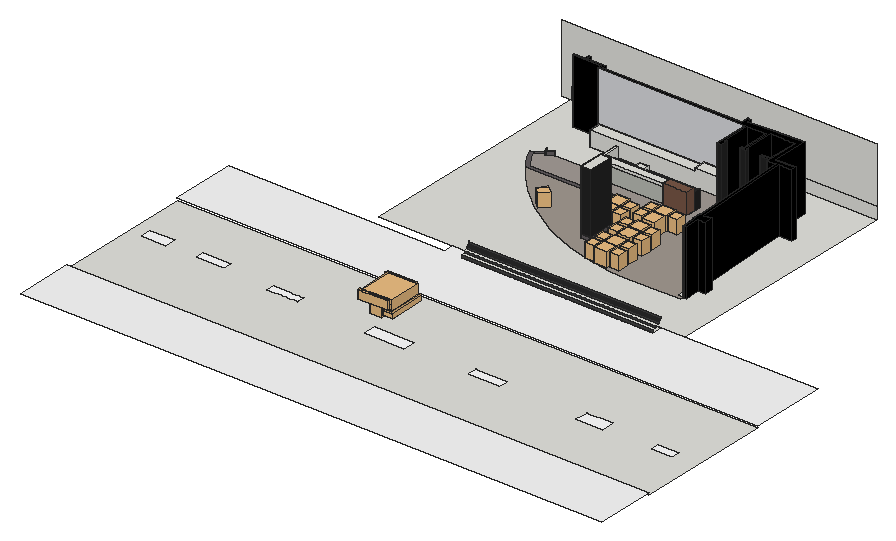
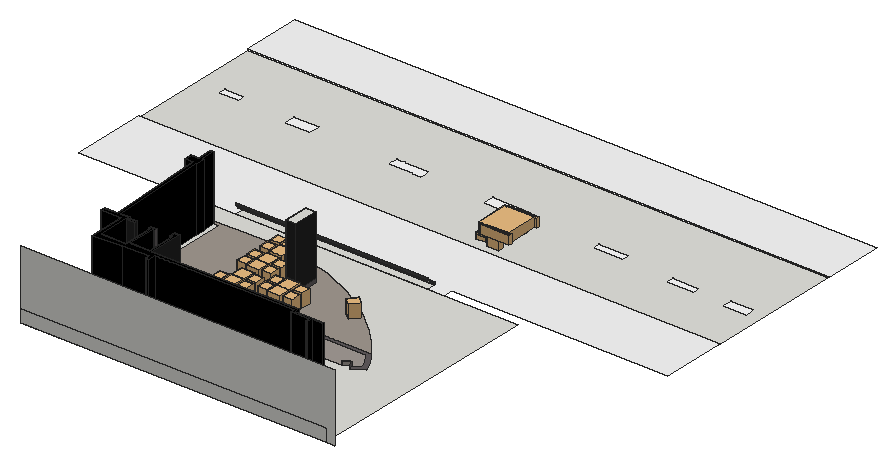
# SketchUp Ruby script. Lengths in inches.
U = 1.inch
M = Sketchup.active_model
def pt(a) = Geom::Point3d.new(a.map { |v| v * U })
def face(e, loops, mat)
  f = e.add_face(loops[0].map { |a| pt(a) })
  loops[1..].each { |l| e.add_face(l.map { |a| pt(a) }).erase! }
  f.material = f.back_material = mat if mat
  f
end
# faces: each face lists its corners as indices into pts; further lists are holes
def faces(e, pts, list, mat = nil) = list.each { |f| face(e, (f[0].is_a?(Array) ? f : [f]).map { |l| l.map { |i| pts[i] } }, mat) }
# xy, xz, yz: faces in a plane at the given z, y or x. An outline is a flat list of corners, or four numbers for a rectangle; further outlines are holes
def ring(l) = l.size == 4 ? [[l[0], l[1]], [l[2], l[1]], [l[2], l[3]], [l[0], l[3]]] : l.each_slice(2).to_a
def flat(e, list, mat, &to3) = list.each { |f| face(e, (f[0].is_a?(Array) ? f : [f]).map { |l| ring(l).map { |u, v| to3.(u, v) } }, mat) }
def xy(e, z, list, mat = nil) = flat(e, list, mat) { |x, y| [x, y, z] }
def xz(e, y, list, mat = nil) = flat(e, list, mat) { |x, z| [x, y, z] }
def yz(e, x, list, mat = nil) = flat(e, list, mat) { |y, z| [x, y, z] }
def lines(e, pts, list) = list.each { |a, b| e.add_line(pt(pts[a]), pt(pts[b])) }
# prism: a flat outline (further loops are holes) pulled along v
def prism(e, loops, v, mat = nil)
  f = face(e, loops, mat); d = Geom::Vector3d.new(v.map { |x| x * U })
  f.pushpull(f.normal.samedirection?(d) ? d.length : -d.length)
end
def box(e, o, s, mat = nil) = prism(e, [[o, [o[0] + s[0], o[1], o[2]], [o[0] + s[0], o[1] + s[1], o[2]], [o[0], o[1] + s[1], o[2]]]], [0, 0, s[2]], mat)
def at(x, y, z, deg = 0) = Geom::Transformation.translation(pt([x, y, z])) * Geom::Transformation.rotation(ORIGIN, Z_AXIS, deg.degrees)
def axes(o, x, y, z) = Geom::Transformation.new([*x, 0, *y, 0, *z, 0, *pt(o).to_a, 1])
def part(name) = M.definitions.add(name)
# library, detail: a bought-in or finely detailed component or shape, given as its bounding box
def library(name, o, s) = part(name).tap { |d| box(d.entities, o, s) }
def detail(e, o, s) = box(e.add_group.entities, o, s)
def put(e, d, t, mat = nil) = e.add_instance(d, t).tap { |i| i.material = mat if mat }
def group(e, t, mat = nil) = e.add_group.tap { |g| g.transformation = t; g.material = mat if mat }.entities
root = M.entities
M.materials.add("Biselado").color = [218, 219, 223]
M.materials.add("Color_").color = [255, 255, 255]
M.materials.add("Concrete").color = [186, 188, 181]
M.materials.add("Floor board2").color = [119, 86, 70]
M.materials.add("Plastic Black ").color = [43, 43, 43]
M.materials.add("Screen Shot 2014-10-30 at 12.13.07").color = [162, 155, 149]
M.materials.add("Sophie_Shoes2").color = [35, 35, 35]
M.materials.add("Sophie_Skirt").color = [0, 0, 0]
M.materials.add("Stain").color = [141, 140, 139]
M.materials.add("Untitsled-1").color = [96, 91, 93]
M.materials.add("Wood_Grain_Dark").color = [51, 47, 43]
M.materials.add("[0132_LightGray]").color = [169, 169, 169]
M.materials.add("[Color_000]").color = [255, 255, 255]
M.materials.add("[Granite Dark Gray]").color = [69, 68, 68]
M.materials.add("[Tile Grey]").color = [249, 249, 249]
M.materials.add("s500 white").color = [237, 237, 230]
M.materials.add("s600").color = [22, 22, 22]
M.materials.add("t_planksnew0027_5_l_seamless_298 copy").color = [161, 153, 144]
c1 = library("Group\#661",[0,74.4,0],[63.33,6.34,17.85])
c2 = library("Car wheel",[-30.53,-13.73,-29.67],[182.47,72.82,182.83])
c3 = library("Group\#641",[0,0,0],[63.89,71.13,20.26])
c4 = library("ch24 wishbone chair by Carl Hansen & Son",[0,0,0],[21.1,19.68,29.02])
c5 = part("Group\#651")
p = [[17.05,0,0.12],[10.76,0.83,0.14],[10.77,0.78,0],[8.125,1.26,0.14],[7.82,1.25,0],[5.66,2.14,0],
  [5.93,2.16,0.13],[4.78,3.14,0.17],[4.32,3.23,0],[3.41,4.89,0],[3.73,4.98,0.17],[1.67,12.39,0],
  [2,12.39,0.17],[0,22.05,0],[0.34,21.8125,0.17],[1.49,22.05,0.22],[16.1,0.375,0.31],[17.15,0.01,0.31],
  [14.125,0.92,0.31],[11.23,1.28,0.31],[8.51,1.62,0.31],[5.54,2.89,0.31],[5.22,3.53,0.31],[4.82,5.07,0.31],
  [3.125,12.39,0.31],[1.65,21.85,0.31]]
faces(c5.entities,p,[[0,1,2],[2,3,4],[3,2,1],[5,4,6],[6,4,3],[7,8,5],[7,5,6],[9,7,10],
  [7,9,8],[11,9,12],[12,9,10],[13,11,14],[14,11,12],[14,15,13],[16,1,17],[1,0,17],
  [1,16,18],[19,3,1],[19,1,18],[3,20,6],[3,19,20],[6,20,21],[21,7,6],[22,7,21],
  [10,7,23],[22,23,7],[24,12,10],[23,24,10],[14,12,25],[24,25,12],[14,25,15]],"[0132_LightGray]")
c6 = library("Component\#54",[-0.14,0,-0.04],[12.61,20.03,8.76])
c7 = library("Group\#643",[0,0,0],[21.93,78.33,4.58])
c8 = library("Group\#650",[0,0,0],[20.12,77.4,9.12])
c9 = library("Group\#658",[0,0,0],[7.9,66.99,3.86])
c10 = part("Untitled (5)")
xy(c10.entities,0,[[[158.81,26.5625,306.06,993.3125],[226.57,518.17,239.57,583.92],[225.28,357.51,237.28,411.51],[222.61,182.28,236.36,226.53],[239.71,931.55,251.46,972.3],[233.64,703.93,242.14,755.18],[240.05,835.03,248.8,880.53],[222.04,66.5,231.29,100.5]]])
xy(c10.entities,0,[[222.04,66.5,231.29,100.5],[222.61,182.28,236.36,226.53],[225.28,357.51,237.28,411.51],[226.57,518.17,239.57,583.92],[233.64,703.93,242.14,755.18],
  [240.05,835.03,248.8,880.53],[239.71,931.55,251.46,972.3]],"Color_")
c11 = library("Square table",[5.01,5.91,-0.2],[27.56,27.56,29.53])
xy(root,-20.5,[[3028.45,559.875,3440.34,581.125],[2834.69,581.125,3491.44,1096.5]])
xy(root,-20.5,[[2527.87,419.4375,3778.5,419.4375,3778.5,581.125,3440.34,581.125,3440.34,559.875,3028.45,559.875,3028.45,581.125,2993.46,581.125,2993.46,559.875,2527.87,559.875]],"[Tile Grey]")
xy(root,-20.25,[[2527.87,0,3778.5,126.25]],"[Tile Grey]")
xy(root,-15.38,[[3028.45,559.875,3440.34,568.25]])
xy(root,-10.73,[[3028.45,568.25,3440.34,575.4375]])
xy(root,-6.62,[[3028.45,575.4375,3440.34,578]])
xy(root,-3.61,[[3028.45,578,3440.34,580.3125]])
xz(root,559.875,[[3028.45,-20.5,3440.34,-15.38]],"[Granite Dark Gray]")
xz(root,568.25,[[3028.45,-15.38,3440.34,-10.73]],"[Granite Dark Gray]")
xz(root,575.4375,[[3028.45,-10.73,3440.34,-6.62]],"[Granite Dark Gray]")
xz(root,578,[[3028.45,-6.62,3440.34,-3.61]],"[Granite Dark Gray]")
xz(root,580.3125,[[3028.45,-3.61,3440.34,1.19]],"[Granite Dark Gray]")
xz(root,1096.5,[[2814.94,-20.5,2814.94,126,3491.44,126,3491.44,6,2834.69,6,2834.69,-20.5],[2834.69,-20.5,3491.44,6]])
yz(root,3028.45,[[578,-6.62,581.125,-3.61],[580.3125,-3.61,581.125,1.19]])
p = [[3061.4375,322.92,0.24],[3061.4375,322.92,0.29],[3037.61,365.74,-9.8],[3037.48,365.73,-9.67],[3037.1875,403.93,-9.8],[3037.05,403.92,-9.67]]
lines(root,p,[[0,1],[2,3],[4,5]])
put(root,c1,axes([3062.39,318.93,-4.37],[-0.99994,-0.01119,0],[-0.01119,0.99994,0],[0,0,1]))
put(root,c1,at(3061.49,399.66,-4.37,-179.359))
put(root,c2,axes([3043.5,395.9,-19.76],[-0.14272,-0.0016,0],[0.0018,-0.16111,0],[0,0,0.14273]))
put(root,c2,axes([3044.33,322.28,-19.76],[-0.14272,-0.0016,0],[-0.0018,0.16111,0],[0,0,0.14273]))
put(root,c3,at(3067.45,394.92,-5.53,-179.359))
put(root,c4,axes([3031.75,755.79,0],[0.63382,0.77348,0],[0.77348,-0.63382,0],[0,0,1]))
put(root,c5,at(3066.33,398.45,-4.68,-179.359),"s600")
put(root,c6,at(3064.43,397.01,-3.93,-179.359))
put(root,c5,axes([3067.2,320.25,-4.68],[-0.99994,-0.01119,0],[-0.01119,0.99994,0],[0,0,1]),"s600")
put(root,c6,axes([3065.27,321.65,-3.93],[-0.99994,-0.01119,0],[-0.01119,0.99994,0],[0,0,1]))
put(root,c7,at(3070.37,398.56,-8.95,-179.359))
put(root,c8,at(3070.4375,398.09,-18.05,-179.359),"s600")
g1 = group(root,at(3064.73,393.36,-4.37,-179.359))
p = [[1.7,7.17,1.16],[1.47,7.32,0],[3.4,0,1.16],[3.17,0,0],[0.28,16.38,1.16],[0,16.77,0],
  [0.28,51.68,1.16],[1.47,60.75,0],[0,51.29,0],[1.7,60.89,1.16],[3.4,68.07,1.16],[3.17,68.06,0]]
faces(g1,p,[[0,1,2],[3,2,1],[4,1,0],[1,4,5],[6,7,8],[7,6,9],[7,9,10],[10,11,7]],"s500 white")
put(root,c9,at(3069.3125,392.875,-15.46,-179.359),"s600")
g2 = group(root,at(3122.24,896.18,31.5))
xy(g2,-31.5,[[0,19.69,18.11,26.38]])
xy(g2,0,[[[0,0,18.11,19.69],[1.09,8.35,17.09,13.35]]])
xy(g2,3.9375,[[[0,0,18.11,26.38],[1.09,8.35,17.09,13.35]]])
xz(g2,0,[[0,0,18.11,3.9375]])
xz(g2,8.35,[[1.09,0,17.09,3.9375]])
xz(g2,13.35,[[1.09,0,17.09,3.9375]])
xz(g2,19.69,[[0,-31.5,18.11,0]])
xz(g2,26.38,[[0,-31.5,18.11,3.9375]])
yz(g2,0,[[19.69,-31.5,19.69,0,0,0,0,3.9375,26.38,3.9375,26.38,-31.5]])
yz(g2,1.09,[[8.35,0,13.35,3.9375]])
yz(g2,17.09,[[8.35,0,13.35,3.9375]])
yz(g2,18.11,[[19.69,-31.5,26.38,-31.5,26.38,3.9375,0,3.9375,0,0,19.69,0]])
g3 = group(root,at(2791.37,624.35,0))
xy(g3,0,[[190.59,338.75,502.63,364.34]],"Stain")
xy(g3,31.5,[[190.59,338.75,416.02,364.34]])
xy(g3,37.4,[[416.02,338.75,502.63,364.34]])
xz(g3,338.75,[[190.59,0,502.63,0,502.63,37.4,416.02,37.4,416.02,31.5,190.59,31.5]])
xz(g3,364.34,[[190.59,0,190.59,31.5,416.02,31.5,416.02,37.4,502.63,37.4,502.63,0]],"Stain")
yz(g3,190.59,[[338.75,0,364.34,31.5]],"Stain")
yz(g3,416.02,[[338.75,31.5,364.34,37.4]])
yz(g3,502.63,[[338.75,0,364.34,37.4]],"Stain")
put(root,c4,axes([3149.53,792.13,0],[0.00287,-1,0],[-1,-0.00287,0],[0,0,1]))
put(root,c4,axes([3149.53,819.14,0],[0.00287,-1,0],[-1,-0.00287,0],[0,0,1]))
g4 = group(root,at(3074.02,896.18,0))
g5 = group(g4,at(0,0,0))
box(g5,[-5.91,0,0],[163.69,19.69,31.5])
put(root,c10,axes([3812.77,-189.95,-24.3125],[0,1.99109,0],[-1.29,0,0],[0,0,1.29]))
g6 = group(root,at(2911.82,841.06,0),"Untitsled-1")
xy(g6,0,[[30.66,0,22.97,10.41,13.17,25.17,0,47.23,25.07,61.99,28.66,54.97,10.82,44.46,19.84,29.37,29.42,14.93,34.63,7.875,502.55,7.875,502.55,0],[29.6875,52.96,28.66,54.97,25.07,61.99,25.45,62.21,29.03,55.19,29.87,53.55,30.06,53.17],[150.39,55.12,162.2,61.02]])
xy(g6,0,[[34.63,7.875,29.42,14.93,19.84,29.37,10.82,44.46,28.66,54.97,29.6875,52.96,30.06,53.17,43.36,60.59,43.25,60.59,43.25,61.02,150.39,61.02,150.39,55.12,295.57,55.12,295.57,74.8,303.44,74.8,303.44,147.64,382.18,147.64,382.18,74.8,392.39,74.8,392.39,88.58,388.09,88.58,388.09,147.64,428.18,147.64,428.18,88.58,423.88,88.58,423.88,82.68,436.24,82.68,436.24,88.58,434.09,88.58,434.09,153.54,485.64,153.54,485.64,88.58,467.74,88.58,467.74,82.68,480.91,82.68,480.91,79.03,503.34,79.03,503.34,31.5,502.55,31.5,502.55,7.875]],"Screen Shot 2014-10-30 at 12.13.07")
xy(g6,0,[[295.57,74.8,303.44,147.64]],"Untitsled-1")
xy(g6,7.875,[[29.6875,52.96,25.07,61.99,25.45,62.21,29.03,55.19,29.87,53.55,43.25,61.02,43.25,60.59,43.36,60.59]],"Untitsled-1")
xz(g6,60.59,[[43.25,0,43.36,7.875]],"Screen Shot 2014-10-30 at 12.13.07")
yz(g6,43.25,[[60.59,0,61.02,7.875]],"Screen Shot 2014-10-30 at 12.13.07")
p = [[29.6875,52.96,7.875],[25.07,61.99,7.875],[25.07,61.99,0],[28.66,54.97,0],[29.6875,52.96,0],[30.06,53.17,0],
  [43.36,60.59,0],[43.36,60.59,7.875],[29.87,53.55,0],[29.03,55.19,0],[29.03,55.19,7.875],[29.87,53.55,7.875],
  [43.25,61.02,0],[43.25,61.02,7.875],[25.45,62.21,0],[25.45,62.21,7.875],[150.39,55.12,0],[150.39,39.37,0],
  [502.55,0,0],[503.34,0,0],[29.44,55.42,0],[43.45,60.64,0],[25.07,62,0],[502.55,78.21,0],
  [480.91,78.21,0],[480.91,79.03,0],[303.44,147.64,0],[303.44,155.51,0]]
faces(g6,p,[[0,1,2,3,4],[4,5,6,7,0],[8,9,10,11],[9,14,15,10],[14,2,1,15]])
faces(g6,p,[[8,12,13,11]],"Screen Shot 2014-10-30 at 12.13.07")
lines(g6,p,[[16,17],[18,19],[20,9],[6,21],[22,2],[23,24],[24,25],[26,27]])
g7 = group(g6,at(388.09,147.64,0))
xy(g7,0,[[0,-59.06,4.3,-59.06,4.3,-58.62,0.43,-58.62,0.43,-0.43,39.67,-0.43,39.67,-58.62,35.8,-58.62,35.8,-59.06,40.1,-59.06,40.1,0,0,0]],"Screen Shot 2014-10-30 at 12.13.07")
xy(g7,7.875,[[0,-59.06,0,-0.43,0.43,-0.43,0.43,-58.62,4.3,-58.62,4.3,-59.06],[35.8,-59.06,35.8,-58.62,39.67,-58.62,39.67,-0.43,40.1,-0.43,40.1,-59.06]],"Untitsled-1")
xy(g7,47.24,[[0,-0.43,40.1,0]],"Untitsled-1")
xz(g7,-59.06,[[35.8,0,40.1,7.875]],"Screen Shot 2014-10-30 at 12.13.07")
xz(g7,-59.06,[[0,0,4.3,7.875]],"Untitsled-1")
xz(g7,-58.62,[[0.43,0,4.3,7.875],[35.8,0,39.67,7.875]],"Untitsled-1")
xz(g7,-0.43,[[0,7.875,40.1,39.37]],"Screen Shot 2014-10-30 at 12.13.07")
xz(g7,-0.43,[[0.43,0,39.67,7.875],[0,39.37,40.1,47.24]],"Untitsled-1")
yz(g7,0,[[-59.06,0,0,0,0,39.37,-0.43,39.37,-0.43,7.875,-59.06,7.875]],"Screen Shot 2014-10-30 at 12.13.07")
yz(g7,0,[[-0.43,39.37,0,47.24]],"Untitsled-1")
yz(g7,0.43,[[-58.62,0,-0.43,7.875]],"Untitsled-1")
yz(g7,4.3,[[-59.06,0,-58.62,7.875]],"Untitsled-1")
yz(g7,35.8,[[-59.06,0,-58.62,7.875]],"Untitsled-1")
yz(g7,39.67,[[-58.62,0,-0.43,7.875]],"Untitsled-1")
yz(g7,40.1,[[-59.06,0,-59.06,7.875,-0.43,7.875,-0.43,39.37,0,39.37,0,0]],"Screen Shot 2014-10-30 at 12.13.07")
yz(g7,40.1,[[-0.43,39.37,0,47.24]],"Untitsled-1")
g8 = group(g6,at(434.09,153.54,0))
xy(g8,0,[[0,-64.96,2.15,-64.96,2.15,-64.53,0.43,-64.53,0.43,-0.43,51.11,-0.43,51.11,-64.53,33.65,-64.53,33.65,-64.96,51.55,-64.96,51.55,0,0,0]],"Screen Shot 2014-10-30 at 12.13.07")
xy(g8,7.875,[[0,-64.96,0,-0.43,0.43,-0.43,0.43,-64.53,2.15,-64.53,2.15,-64.96],[33.65,-64.96,33.65,-64.53,51.11,-64.53,51.11,-0.43,51.55,-0.43,51.55,-64.96]],"Untitsled-1")
xy(g8,47.24,[[0,-0.43,51.55,0]],"Untitsled-1")
xz(g8,-64.96,[[0,0,2.15,7.875],[33.65,0,51.55,7.875]],"Untitsled-1")
xz(g8,-64.53,[[0.43,0,2.15,7.875],[33.65,0,51.11,7.875]],"Untitsled-1")
xz(g8,-0.43,[[0,7.875,51.55,39.37]],"Screen Shot 2014-10-30 at 12.13.07")
xz(g8,-0.43,[[0.43,0,51.11,7.875],[0,39.37,51.55,47.24]],"Untitsled-1")
xz(g8,0,[[40.1,0,51.55,39.37]],"Screen Shot 2014-10-30 at 12.13.07")
xz(g8,0,[[40.1,39.37,51.55,47.24]],"Untitsled-1")
yz(g8,0,[[-64.96,0,0,0,0,39.37,-0.43,39.37,-0.43,7.875,-64.96,7.875]],"Screen Shot 2014-10-30 at 12.13.07")
yz(g8,0,[[-0.43,39.37,0,47.24]],"Untitsled-1")
yz(g8,0.43,[[-64.53,0,-0.43,7.875]],"Untitsled-1")
yz(g8,2.15,[[-64.96,0,-64.53,7.875]],"Untitsled-1")
yz(g8,33.65,[[-64.96,0,-64.53,7.875]],"Untitsled-1")
yz(g8,51.11,[[-64.53,0,-0.43,7.875]],"Untitsled-1")
yz(g8,51.55,[[-64.96,0,-64.96,7.875,-0.43,7.875,-0.43,39.37,0,39.37,0,0]],"Screen Shot 2014-10-30 at 12.13.07")
yz(g8,51.55,[[-0.43,39.37,0,47.24]],"Untitsled-1")
put(root,c11,at(3186.21,762.18,0,89.836))
put(root,c11,at(3186.21,790.25,0,89.836))
g9 = group(root,at(3165.33,710.08,0))
xy(g9,0,[[-0.59,-0.59,22.24,53.74]])
xy(g9,7.875,[[-0.59,-0.59,22.24,0],[-0.59,0,0,53.15],[21.65,0,22.24,53.15],[-0.59,53.15,22.24,53.74]],"Untitsled-1")
xy(g9,137.44,[[0,0,21.65,53.15]])
xz(g9,-0.59,[[-0.59,0,22.24,7.875]],"Untitsled-1")
xz(g9,0,[[0,7.875,21.65,137.44]],"Sophie_Shoes2")
xz(g9,53.15,[[0,7.875,21.65,137.44]],"Sophie_Shoes2")
xz(g9,53.74,[[-0.59,0,22.24,7.875]],"Untitsled-1")
yz(g9,-0.59,[[-0.59,0,53.74,7.875]],"Untitsled-1")
yz(g9,0,[[0,7.875,53.15,137.44]],"Sophie_Shoes2")
yz(g9,21.65,[[0,7.875,53.15,137.44]],"Sophie_Shoes2")
yz(g9,22.24,[[-0.59,0,53.74,7.875]],"Untitsled-1")
g10 = group(root,at(2915.67,657.41,0))
xy(g10,0,[[511.73,0,511.7,0.79,510.27,31.46,508.31,31.46,507.48,49.07,509.45,49.07,499.49,263.4,481.79,262.65,481.79,265.89,463.89,265.89,463.89,272.23,481.79,272.23,481.79,337.19,430.24,337.19,430.24,272.23,432.39,272.23,432.39,265.89,420.03,265.89,420.03,272.23,424.33,272.23,424.33,331.29,384.24,331.29,384.24,272.23,388.54,272.23,388.54,258.02,377.9,258.02,377.9,331.29,62.06,331.29,62.06,341.13,1.14,341.13,0,345.07,25.02,345.07,25.02,355.33,28.95,355.33,28.95,347.03,67.96,347.03,67.96,339.16,365.84,339.16,365.84,355.33,373.72,355.33,373.72,346.57,430.24,349.18,491.63,352.02,491.63,272.99,534.09,274.79,534.09,264.94,507.35,263.81,517.3125,49.53,534.09,50.31,534.09,32.57,518.14,31.83,519.6,0.37,514.8125,0]],"Sophie_Skirt")
xy(g10,7.875,[[377.9,258.02,378.33,331.29],[378.33,258.02,388.54,258.45],[420.03,265.89,432.39,266.33],[463.89,265.89,481.79,266.33]],"Untitsled-1")
xy(g10,137.8,[[511.73,0,514.8125,0,519.6,0.37,518.14,31.83,534.09,32.57,534.09,50.31,517.3125,49.53,507.35,263.81,534.09,264.94,534.09,274.79,491.63,272.99,491.63,352.02,430.24,349.18,373.72,346.57,373.72,355.33,365.84,355.33,365.84,339.16,67.96,339.16,67.96,347.03,28.95,347.03,28.95,355.33,25.02,355.33,25.02,345.07,0,345.07,1.14,341.13,62.06,341.13,62.06,331.29,378.33,331.29,378.33,258.45,388.54,258.45,388.54,272.23,384.24,272.23,384.24,331.29,424.33,331.29,424.33,272.23,420.03,272.23,420.03,266.33,432.39,266.33,432.39,272.23,430.24,272.23,430.24,337.19,481.79,337.19,481.79,272.23,463.89,272.23,463.89,266.33,481.79,266.33,481.79,262.65,499.49,263.4,509.45,49.07,507.48,49.07,508.31,31.46,510.27,31.46,511.7,0.79]],"Sophie_Skirt")
xz(g10,0,[[511.73,0,514.8125,137.8]],"Sophie_Skirt")
xz(g10,31.46,[[508.31,0,510.27,137.8]],"Sophie_Skirt")
xz(g10,49.07,[[507.48,0,509.45,137.8]],"Sophie_Skirt")
xz(g10,258.02,[[377.9,0,388.54,7.875]],"Untitsled-1")
xz(g10,258.45,[[378.33,7.875,388.54,137.8]],"Sophie_Shoes2")
xz(g10,265.89,[[420.03,0,432.39,7.875],[463.89,0,481.79,7.875]],"Untitsled-1")
xz(g10,266.33,[[420.03,7.875,432.39,137.8],[463.89,7.875,481.79,137.8]],"Sophie_Shoes2")
xz(g10,272.23,[[384.24,0,388.54,137.8],[420.03,0,424.33,137.8],[430.24,0,432.39,137.8],[463.89,0,481.79,137.8]],"Sophie_Shoes2")
xz(g10,331.29,[[62.06,0,377.9,0,377.9,7.875,378.33,7.875,378.33,137.8,62.06,137.8]],"Biselado")
xz(g10,331.29,[[384.24,0,424.33,137.8]],"Sophie_Skirt")
xz(g10,337.19,[[430.24,0,481.79,137.8]],"Sophie_Skirt")
xz(g10,339.16,[[67.96,0,365.84,137.8]],"Sophie_Skirt")
xz(g10,341.13,[[1.14,0,62.06,137.8]],"Sophie_Skirt")
xz(g10,345.07,[[0,0,25.02,137.8]],"Sophie_Skirt")
xz(g10,347.03,[[28.95,0,67.96,137.8]],"Sophie_Skirt")
xz(g10,355.33,[[25.02,0,28.95,137.8],[365.84,0,373.72,137.8]],"Sophie_Skirt")
yz(g10,25.02,[[345.07,0,355.33,137.8]],"Sophie_Skirt")
yz(g10,28.95,[[347.03,0,355.33,137.8]],"Sophie_Skirt")
yz(g10,62.06,[[331.29,0,341.13,137.8]],"Sophie_Skirt")
yz(g10,67.96,[[339.16,0,347.03,137.8]],"Sophie_Skirt")
yz(g10,365.84,[[339.16,0,355.33,137.8]],"Sophie_Skirt")
yz(g10,373.72,[[346.57,0,355.33,137.8]],"Sophie_Skirt")
yz(g10,377.9,[[258.02,0,331.29,7.875]],"Untitsled-1")
yz(g10,378.33,[[258.45,7.875,331.29,137.8]],"Sophie_Shoes2")
yz(g10,384.24,[[272.23,0,331.29,137.8]],"Sophie_Skirt")
yz(g10,388.54,[[258.02,0,272.23,0,272.23,137.8,258.45,137.8,258.45,7.875,258.02,7.875]],"Sophie_Shoes2")
yz(g10,420.03,[[265.89,0,265.89,7.875,266.33,7.875,266.33,137.8,272.23,137.8,272.23,0]],"Untitsled-1")
yz(g10,424.33,[[272.23,0,331.29,137.8]],"Sophie_Skirt")
yz(g10,430.24,[[272.23,0,337.19,137.8]],"Sophie_Skirt")
yz(g10,432.39,[[265.89,0,272.23,0,272.23,137.8,266.33,137.8,266.33,7.875,265.89,7.875]],"Sophie_Shoes2")
yz(g10,463.89,[[265.89,0,265.89,7.875,266.33,7.875,266.33,137.8,272.23,137.8,272.23,0]],"Sophie_Shoes2")
yz(g10,481.79,[[262.65,0,262.65,137.8,266.33,137.8,266.33,7.875,265.89,7.875,265.89,0],[272.23,0,337.19,137.8]],"Sophie_Skirt")
yz(g10,491.63,[[272.99,0,352.02,137.8]],"Sophie_Skirt")
yz(g10,534.09,[[32.57,0,50.31,137.8],[264.94,0,274.79,137.8]],"Sophie_Skirt")
p = [[511.7,0.79,0],[511.73,0,0],[511.73,0,137.8],[511.7,0.79,137.8],[514.8125,0,0],[519.6,0.37,0],
  [519.6,0.37,137.8],[514.8125,0,137.8],[518.14,31.83,0],[518.14,31.83,137.8],[510.27,31.46,0],[510.27,31.46,137.8],
  [507.48,49.07,0],[508.31,31.46,0],[508.31,31.46,137.8],[507.48,49.07,137.8],[534.09,32.57,0],[534.09,32.57,137.8],
  [499.49,263.4,0],[509.45,49.07,0],[509.45,49.07,137.8],[499.49,263.4,137.8],[517.3125,49.53,0],[507.35,263.81,0],
  [507.35,263.81,137.8],[517.3125,49.53,137.8],[534.09,50.31,0],[534.09,50.31,137.8],[481.79,262.65,0],[481.79,262.65,137.8],
  [534.09,264.94,0],[534.09,264.94,137.8],[534.09,274.79,0],[491.63,272.99,0],[491.63,272.99,137.8],[534.09,274.79,137.8],
  [0,345.07,0],[1.14,341.13,0],[1.14,341.13,137.8],[0,345.07,137.8],[430.24,349.18,0],[373.72,346.57,0],
  [373.72,346.57,137.8],[430.24,349.18,137.8],[491.63,352.02,0],[491.63,352.02,137.8]]
faces(g10,p,[[0,1,2,3],[4,5,6,7],[5,8,9,6],[10,0,3,11],[12,13,14,15],[8,16,17,9],[18,19,20,21],[22,23,24,25],
  [26,22,25,27],[28,18,21,29],[23,30,31,24],[32,33,34,35],[36,37,38,39],[40,41,42,43],[44,40,43,45]],"Sophie_Skirt")
g11 = group(g10,at(146.54,223.02,0))
xy(g11,0,[[0,0,0,51.18,5.91,51.18,5.91,16.93,145.18,16.93,145.18,6.69,5.91,6.69,5.91,0]],"Concrete")
xy(g11,37.4,[[5.91,0,145.18,6.69]])
xy(g11,43.31,[[0,0,145.18,0,145.18,16.93,5.91,16.93,5.91,51.18,0,51.18]])
xz(g11,0,[[0,0,5.91,0,5.91,37.4,145.18,37.4,145.18,43.31,0,43.31]])
xz(g11,6.69,[[5.91,36.8125,6.5,36.8125,10.63,37.4,5.91,37.4]])
xz(g11,6.69,[[5.91,0,5.91,36.8125,6.5,36.8125,10.63,37.4,145.18,37.4,145.18,0]],"Concrete")
xz(g11,16.93,[[5.91,0,145.18,43.31]],"[Color_000]")
xz(g11,51.18,[[0,0,5.91,43.31]],"Concrete")
yz(g11,0,[[0,0,51.18,43.31]])
yz(g11,5.91,[[0,0,6.69,37.4],[16.93,0,51.18,43.31]])
yz(g11,145.18,[[6.69,0,16.93,0,16.93,43.31,0,43.31,0,37.4,6.69,37.4]],"Concrete")
p = [[190.45,16.14,0],[190.45,15.75,0],[169.59,16.14,0],[169.59,15.75,0]]
lines(g11,p,[[0,1],[2,3]])
g12 = group(root,at(2942.48,648.17,0),"t_planksnew0027_5_l_seamless_298 copy")
xy(g12,0,[[429.35,0,354.79,0.42,331.3,2.55,319.24,4.03,295.95,7.5625,272.9,12.11,229.52,24.41,206.75,33.49,183.99,42.57,173.49,47.99,162.94,53.43,103.01,90.75,94.03,97,85.51,104.03,76.98,111.05,63.55,122.79,50.29,134.84,37.79,147.5,24.1875,162.86,7,183.74,0,192.89,472.68,192.89,472.68,9.29,486.38,9.29,486.38,1.89]],"t_planksnew0027_5_l_seamless_298 copy")
put(root,c4,at(3183.1,819.14,0,-90.164))
put(root,c4,at(3183.1,792.13,0,-90.164))
put(root,c4,at(3232.59,724,0,89.836))
put(root,c4,at(3232.59,689.04,0,89.836))
put(root,c4,at(3232.59,751,0,89.836))
put(root,c4,at(3232.59,660.73,0,89.836))
put(root,c4,at(3232.59,790.81,0,89.836))
put(root,c4,at(3232.59,817.82,0,89.836))
g13 = group(root,at(3207.38,877.67,0))
g14 = group(g13,at(0,0,0))
xy(g14,1.97,[[24.41,37.01,25.2,37.4],[25.2,37.01,48.23,37.4]],"Sophie_Shoes2")
xy(g14,1.97,[[48.23,37.01,50,38.1875]],"Wood_Grain_Dark")
xy(g14,2.76,[[0,0,51.18,10.24],[25.2,19.69,48.23,37.4]],"Plastic Black ")
xy(g14,2.76,[[50,10.24,51.18,19.25]],"Wood_Grain_Dark")
xy(g14,13.58,[[25.2,19.69,48.23,37.01]],"Plastic Black ")
xy(g14,14.37,[[25.2,19.69,48.23,37.01]],"Plastic Black ")
xy(g14,25.98,[[25.2,19.69,48.23,37.4]],"Plastic Black ")
xy(g14,26.77,[[25.2,19.69,48.23,19.69,48.23,22.83,47.44,22.83,47.44,37.4,25.2,37.4]],"Plastic Black ")
xy(g14,27.6875,[[27.68,18.11,45.43,19.69]])
xy(g14,30.71,[[25.2,22.83,47.44,37.4]],"Plastic Black ")
xy(g14,31.23,[[27.68,18.11,45.43,19.69]])
xy(g14,31.5,[[24.41,19.69,25.2,19.69,25.2,22.83,48.23,22.83,48.23,37.4,24.41,37.4]],"Plastic Black ")
xy(g14,35.93,[[24.41,19.25,50,19.25,50,38.1875,48.23,38.1875,48.23,19.69,24.41,19.69]],"Sophie_Shoes2")
xy(g14,35.93,[[0,19.25,24.41,19.69]],"[Color_000]")
xy(g14,46.0625,[[0,0,51.18,19.25]],"Floor board2")
xz(g14,0,[[0,2.76,51.18,46.0625]],"Floor board2")
xz(g14,10.24,[[0,0,50,2.76]],"Plastic Black ")
xz(g14,18.11,[[27.68,27.6875,45.43,31.23]])
xz(g14,19.25,[[50,2.76,50,35.93,0,35.93,0,46.0625,51.18,46.0625,51.18,2.76]],"Floor board2")
xz(g14,19.69,[[25.2,2.76,48.23,13.58],[25.2,13.58,48.23,14.37],[25.2,14.37,48.23,25.98]],"Plastic Black ")
xz(g14,19.69,[[[25.2,26.77,25.2,31.5,24.41,31.5,24.41,35.93,48.23,35.93,48.23,26.77],[27.68,27.6875,45.43,31.23]]],"Sophie_Shoes2")
xz(g14,19.69,[[0,0,24.41,35.93]],"[Color_000]")
xz(g14,22.83,[[47.44,26.77,48.23,26.77,48.23,31.5,25.2,31.5,25.2,30.71,47.44,30.71]],"Plastic Black ")
xz(g14,37.01,[[25.2,13.58,48.23,14.37]],"Plastic Black ")
xz(g14,37.01,[[24.41,0,50,1.97]],"Sophie_Shoes2")
xz(g14,37.4,[[[24.41,1.97,24.41,31.5,48.23,31.5,48.23,25.98,25.2,25.98,25.2,2.76,48.23,2.76,48.23,1.97],[25.2,26.77,47.44,30.71]]],"Sophie_Shoes2")
xz(g14,38.1875,[[48.23,1.97,50,35.93]],"Plastic Black ")
yz(g14,0,[[10.24,0,10.24,2.76,0,2.76,0,46.0625,19.25,46.0625,19.25,0]],"Floor board2")
yz(g14,0,[[19.25,0,19.69,35.93]],"[Color_000]")
yz(g14,24.41,[[19.69,0,19.69,31.5,37.4,31.5,37.4,1.97,37.01,1.97,37.01,0]],"Plastic Black ")
yz(g14,25.2,[[19.69,2.76,37.4,13.58],[19.69,13.58,37.01,14.37],[19.69,14.37,37.4,25.98],[19.69,26.77,37.4,26.77,37.4,30.71,22.83,30.71,22.83,31.5,19.69,31.5]],"Plastic Black ")
yz(g14,25.2,[[37.01,13.58,37.4,14.37]],"Sophie_Shoes2")
yz(g14,27.68,[[18.11,27.6875,19.69,31.23]])
yz(g14,45.43,[[18.11,27.6875,19.69,31.23]])
yz(g14,47.44,[[22.83,26.77,37.4,30.71]],"Plastic Black ")
yz(g14,48.23,[[37.4,1.97,37.4,2.76,19.69,2.76,19.69,13.58,37.01,13.58,37.01,14.37,19.69,14.37,19.69,25.98,37.4,25.98,37.4,31.5,22.83,31.5,22.83,26.77,19.69,26.77,19.69,35.93,38.1875,35.93,38.1875,1.97],[19.69,13.58,37.01,14.37]],"Plastic Black ")
yz(g14,50,[[10.24,0,37.01,0,37.01,1.97,38.1875,1.97,38.1875,35.93,19.25,35.93,19.25,2.76,10.24,2.76]],"Sophie_Shoes2")
yz(g14,51.18,[[0,2.76,19.25,46.0625]],"Floor board2")
p = [[24.41,18.5,46.0625],[24.41,18.5,46.16],[0,8.86,37.4],[0,10.24,37.4]]
lines(g14,p,[[0,1],[2,3]])
put(root,c11,at(3229.48,717.93,0,-90.164))
put(root,c11,at(3229.48,780.96,0,-90.164))
put(root,c11,at(3229.48,689.86,0,-90.164))
put(root,c11,at(3229.48,752.89,0,-90.164))
put(root,c11,at(3229.48,847.77,0,-90.164))
put(root,c11,at(3229.48,819.7,0,-90.164))
put(root,c4,axes([3266.16,751,0],[-0.00287,1,0],[1,0.00287,0],[0,0,1]))
put(root,c4,axes([3266.16,724,0],[-0.00287,1,0],[1,0.00287,0],[0,0,1]))
put(root,c4,axes([3266.16,660.73,0],[-0.00287,1,0],[1,0.00287,0],[0,0,1]))
put(root,c4,axes([3266.16,689.04,0],[-0.00287,1,0],[1,0.00287,0],[0,0,1]))
put(root,c4,axes([3266.16,817.82,0],[-0.00287,1,0],[1,0.00287,0],[0,0,1]))
